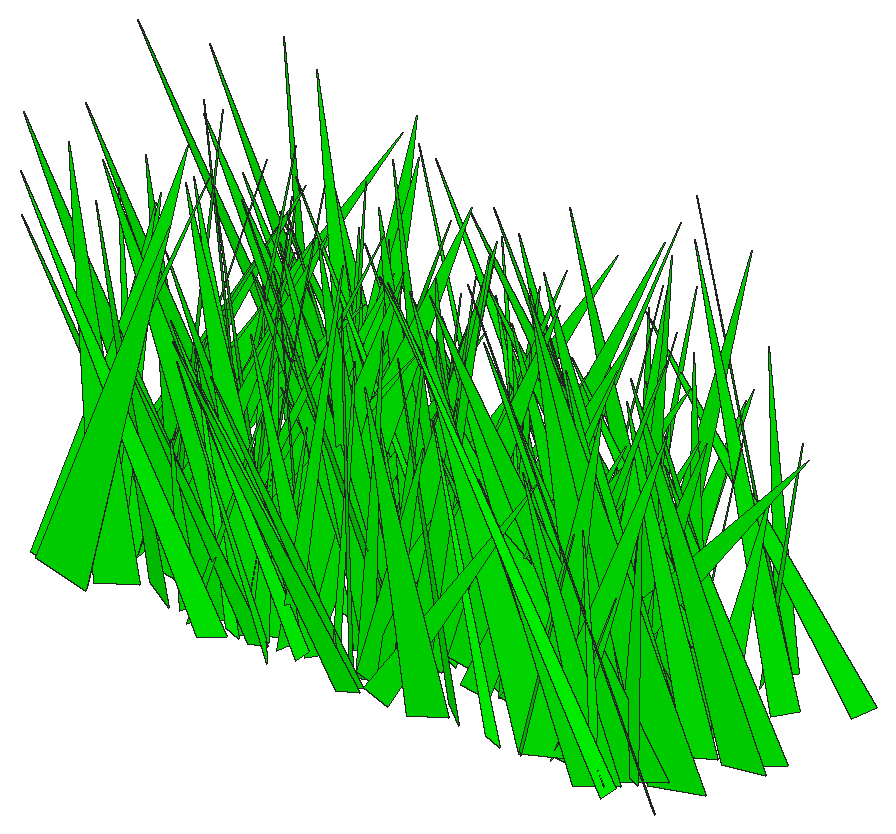
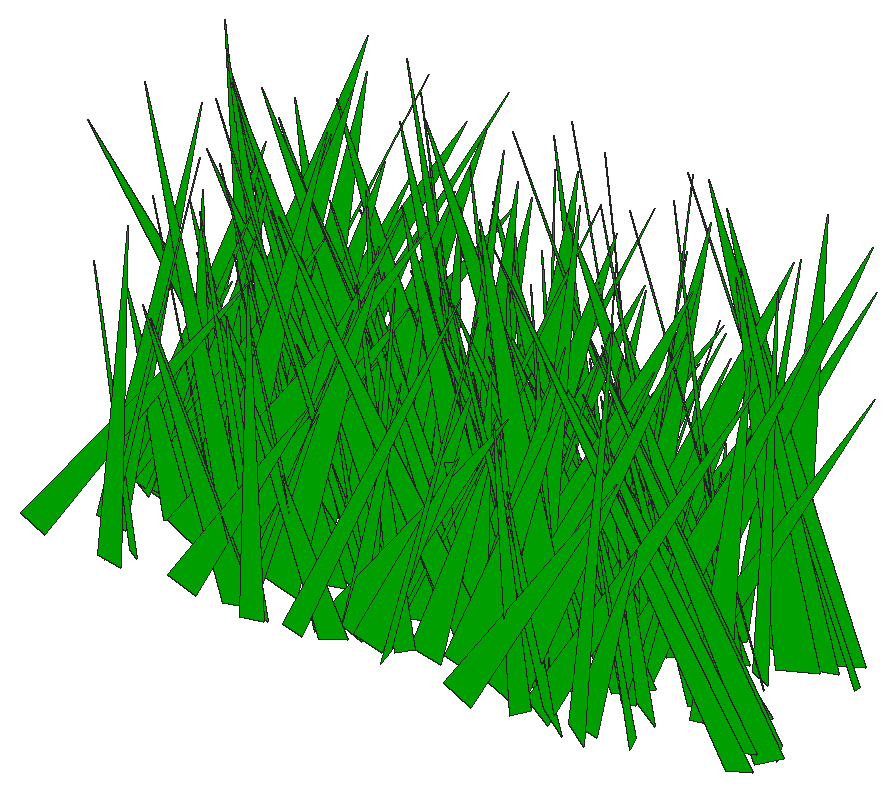
# SketchUp Ruby script. Lengths in inches.
U = 1.inch
M = Sketchup.active_model
def pt(a) = Geom::Point3d.new(a.map { |v| v * U })
def face(e, loops, mat)
  f = e.add_face(loops[0].map { |a| pt(a) })
  loops[1..].each { |l| e.add_face(l.map { |a| pt(a) }).erase! }
  f.material = f.back_material = mat if mat
  f
end
# faces: each face lists its corners as indices into pts; further lists are holes
def faces(e, pts, list, mat = nil) = list.each { |f| face(e, (f[0].is_a?(Array) ? f : [f]).map { |l| l.map { |i| pts[i] } }, mat) }
# xy, xz, yz: faces in a plane at the given z, y or x. An outline is a flat list of corners, or four numbers for a rectangle; further outlines are holes
def ring(l) = l.size == 4 ? [[l[0], l[1]], [l[2], l[1]], [l[2], l[3]], [l[0], l[3]]] : l.each_slice(2).to_a
def flat(e, list, mat, &to3) = list.each { |f| face(e, (f[0].is_a?(Array) ? f : [f]).map { |l| ring(l).map { |u, v| to3.(u, v) } }, mat) }
def xy(e, z, list, mat = nil) = flat(e, list, mat) { |x, y| [x, y, z] }
def xz(e, y, list, mat = nil) = flat(e, list, mat) { |x, z| [x, y, z] }
def yz(e, x, list, mat = nil) = flat(e, list, mat) { |y, z| [x, y, z] }
def lines(e, pts, list) = list.each { |a, b| e.add_line(pt(pts[a]), pt(pts[b])) }
# prism: a flat outline (further loops are holes) pulled along v
def prism(e, loops, v, mat = nil)
  f = face(e, loops, mat); d = Geom::Vector3d.new(v.map { |x| x * U })
  f.pushpull(f.normal.samedirection?(d) ? d.length : -d.length)
end
def box(e, o, s, mat = nil) = prism(e, [[o, [o[0] + s[0], o[1], o[2]], [o[0] + s[0], o[1] + s[1], o[2]], [o[0], o[1] + s[1], o[2]]]], [0, 0, s[2]], mat)
def at(x, y, z, deg = 0) = Geom::Transformation.translation(pt([x, y, z])) * Geom::Transformation.rotation(ORIGIN, Z_AXIS, deg.degrees)
def axes(o, x, y, z) = Geom::Transformation.new([*x, 0, *y, 0, *z, 0, *pt(o).to_a, 1])
def part(name) = M.definitions.add(name)
# library, detail: a bought-in or finely detailed component or shape, given as its bounding box
def library(name, o, s) = part(name).tap { |d| box(d.entities, o, s) }
def detail(e, o, s) = box(e.add_group.entities, o, s)
def put(e, d, t, mat = nil) = e.add_instance(d, t).tap { |i| i.material = mat if mat }
def group(e, t, mat = nil) = e.add_group.tap { |g| g.transformation = t; g.material = mat if mat }.entities
root = M.entities
M.materials.add("[0065_Lime]").color = [0, 255, 0]
c1 = part("fur_instance\#9")
p = [[0.8125,0,1.79],[0.67,-0.02,1.48],[0,-0.11,0],[0,0.11,0]]
faces(c1.entities,p,[[0,1,2,3]])
put(root,c1,axes([48.68,23.55,1.48],[-4.07372,-0.91201,0.20358],[6.33455,-0.56704,-1.2527],[1.43544,-0.08593,6.1059]),"[0065_Lime]")
put(root,c1,axes([51.56,20.1,1.48],[-5.89201,-0.44305,0.24837],[3.10748,-0.79083,1.50424],[-0.61473,0.24881,5.22342]),"[0065_Lime]")
put(root,c1,axes([46.21,23.61,1.48],[6.74369,-0.00029,0.17431],[0.06941,0.89987,-1.72693],[-0.20276,0.29849,5.20647]),"[0065_Lime]")
put(root,c1,axes([52.6875,25.88,1.48],[-7.7799,-0.6017,0.36466],[4.2396,-1.04797,1.90215],[-0.75013,0.31754,6.96855]),"[0065_Lime]")
put(root,c1,axes([51.88,23.01,1.48],[-4.98454,-0.94604,0.09844],[6.66124,-0.68968,1.06821],[-0.98445,0.12331,6.72962]),"[0065_Lime]")
put(root,c1,axes([49.63,19.33,1.48],[5.19849,-0.96659,1.66799],[6.54163,0.78443,1.74286],[-2.95466,0.03608,6.7934]),"[0065_Lime]")
put(root,c1,axes([49.17,20.73,1.48],[-6.82183,0.05565,2.74804],[-1.5285,-1.00055,-1.83157],[3.03877,-0.37835,5.24787]),"[0065_Lime]")
put(root,c1,axes([46.15,24.125,1.48],[6.47814,-0.51925,0.67202],[3.76421,0.85822,-1.78814],[0.41013,0.32493,5.79688]),"[0065_Lime]")
put(root,c1,axes([48.32,19.46,1.48],[-1.28615,1.01519,1.55532],[-7.2535,-0.23522,1.17596],[1.79941,-0.22254,5.85201]),"[0065_Lime]")
put(root,c1,axes([48.63,19.8,1.48],[-3.52804,0.92999,1.4678],[-6.38089,-0.54957,1.52025],[2.51841,-0.08963,5.90809]),"[0065_Lime]")
put(root,c1,axes([47.06,24.2,1.48],[3.35952,0.76991,0.39872],[-5.32449,0.43483,1.54786],[1.38223,-0.19626,4.99344]),"[0065_Lime]")
put(root,c1,axes([46.78,19.58,1.48],[8.93201,0.21826,0.83479],[-1.73967,1.2302,1.53789],[-0.66288,-0.28758,7.21231]),"[0065_Lime]")
put(root,c1,axes([47.96,18.92,1.48],[-2.61508,1.25456,1.37276],[-8.47503,-0.42576,2.3563],[3.27618,-0.09998,7.19117]),"[0065_Lime]")
put(root,c1,axes([53.14,19.56,1.48],[-4.27079,-1.12782,0.92461],[7.91508,-0.54119,2.06895],[-1.75029,0.30458,7.10002]),"[0065_Lime]")
put(root,c1,axes([49.6,25.65,1.48],[4.1549,0.03918,1.15757],[0.34748,0.56226,-1.46292],[-1.40791,0.25439,3.05505]),"[0065_Lime]")
put(root,c1,axes([50.97,24.03,1.48],[-4.48205,-0.3349,0.36033],[2.21663,-0.61916,-1.04063],[0.98144,-0.13104,3.99588]),"[0065_Lime]")
put(root,c1,axes([51.14,25.84,1.48],[0.00797,0.625,0.25599],[-4.29085,0.0131,-0.9836],[-1.21279,-0.04225,3.48166]),"[0065_Lime]")
put(root,c1,axes([53.42,18.66,1.48],[-7.20831,0.54493,0.08946],[-3.85095,-1.00106,-0.97205],[-0.47041,-0.15514,6.58667]),"[0065_Lime]")
put(root,c1,axes([50.88,19.57,1.48],[-6.81332,-0.57827,1.01934],[3.6731,-0.95369,-1.88538],[2.23932,-0.19513,6.19395]),"[0065_Lime]")
put(root,c1,axes([49.39,21.31,1.48],[4.09738,-0.2315,0.5266],[1.45263,0.57084,0.93058],[-1.01151,-0.11797,3.46956]),"[0065_Lime]")
put(root,c1,axes([48.13,18.79,1.48],[0.37992,-1.11269,1.4575],[7.83928,-0.01529,-1.74306],[2.11176,0.25693,6.2084]),"[0065_Lime]")
put(root,c1,axes([51.09,26.22,1.48],[-7.64642,-0.31284,2.79186],[3.21779,-1.09124,1.73359],[2.52646,0.44302,6.2417]),"[0065_Lime]")
put(root,c1,axes([46.45,25.04,1.48],[7.70161,0.7186,0.15562],[-4.98191,1.04168,1.94706],[1.17045,-0.29463,7.26346]),"[0065_Lime]")
put(root,c1,axes([50.32,24.19,1.48],[5.50694,0.53946,0.7244],[-3.39627,0.75869,-1.84981],[-1.99931,0.1971,5.13762]),"[0065_Lime]")
put(root,c1,axes([50.11,20.95,1.48],[8.62522,0.15611,2.42075],[-0.39976,1.25374,-1.76682],[-3.15138,0.26822,6.84963]),"[0065_Lime]")
put(root,c1,axes([53.9,25.77,1.48],[-6.69789,-0.79189,0.81059],[5.71052,-0.9106,1.41088],[-0.37651,0.27607,6.97887]),"[0065_Lime]")
put(root,c1,axes([49.07,20.81,1.48],[8.5082,0.29483,1.00981],[-1.81444,1.18877,-1.51533],[-1.62829,0.21588,6.96508]),"[0065_Lime]")
put(root,c1,axes([49.58,23.01,1.48],[5.62934,0.37435,1.24764],[-3.00109,0.76666,1.25101],[-0.66592,-0.29052,4.90896]),"[0065_Lime]")
put(root,c1,axes([54.51,19.54,1.48],[-2.83101,1.08435,1.40047],[-7.66821,-0.31393,-2.1111],[-1.92679,-0.34384,6.34401]),"[0065_Lime]")
put(root,c1,axes([47.75,22.59,1.48],[4.43363,0.75456,0.40978],[-4.86388,0.51978,2.74705],[2.33055,-0.35067,4.95359]),"[0065_Lime]")
put(root,c1,axes([51.97,19.51,1.48],[2.89859,-0.42098,0.0198],[2.6624,0.36412,1.53792],[-1.37392,-0.18255,3.02197]),"[0065_Lime]")
put(root,c1,axes([50.93,23.875,1.48],[-0.9214,-0.66428,0.38057],[4.40262,-0.14456,-1.40289],[1.78438,0.01367,3.65788]),"[0065_Lime]")
put(root,c1,axes([54.39,20.9,1.48],[-4.60535,-0.60324,0.97308],[4.44191,-0.60177,1.40869],[-0.36068,0.29139,4.92364]),"[0065_Lime]")
put(root,c1,axes([54.92,26.51,1.48],[-3.41391,-0.66832,0.40587],[4.55813,-0.42867,1.71429],[-1.44688,0.22646,4.44291]),"[0065_Lime]")
put(root,c1,axes([50.23,20.58,1.48],[3.70843,-0.68218,0.79021],[4.91564,0.48696,-1.17652],[0.59091,0.23032,4.82796]),"[0065_Lime]")
put(root,c1,axes([51.0625,21.53,1.48],[8.5129,0.07603,1.98454],[0.11365,1.20408,-1.86829],[-2.49646,0.31407,6.68221]),"[0065_Lime]")
put(root,c1,axes([53.85,20.47,1.48],[-6.25726,0.72762,0.42309],[-5.08217,-0.87895,0.92111],[1.12025,0.0767,6.54198]),"[0065_Lime]")
put(root,c1,axes([53.5625,21.07,1.48],[-7.52551,-0.2028,1.95223],[1.84318,-1.08667,0.91837],[2.10853,0.2261,6.16488]),"[0065_Lime]")
put(root,c1,axes([54.66,19.0625,1.48],[-3.79363,-0.52252,0.09486],[3.63146,-0.51499,1.03323],[-0.80852,0.13864,4.19565]),"[0065_Lime]")
put(root,c1,axes([53.5,20.51,1.48],[-8.88237,-0.10563,2.45717],[1.31519,-1.29059,1.28654],[2.82146,0.26906,7.13581]),"[0065_Lime]")
put(root,c1,axes([49.51,21.66,1.48],[4.14624,-1.01049,0.18664],[7.05449,0.56365,-1.43235],[1.41409,0.15094,6.59835]),"[0065_Lime]")
put(root,c1,axes([55.65,23.77,1.48],[1.72035,-1.18418,1.79479],[7.65245,0.35645,3.02737],[-4.16257,0.16588,6.30728]),"[0065_Lime]")
put(root,c1,axes([52.6,21.36,1.48],[-5.25279,0.17933,1.77712],[-0.64661,-0.77908,1.36978],[2.44618,0.17914,4.17818]),"[0065_Lime]")
put(root,c1,axes([55.3,24.21,1.48],[-5.86449,0.56431,0.65677],[-4.087,-0.79274,-1.32174],[-0.27545,-0.25201,5.62841]),"[0065_Lime]")
put(root,c1,axes([52.32,22.48,1.48],[5.06736,-0.33017,0.90518],[1.83122,0.69643,1.72939],[-1.84552,-0.21553,4.2014]),"[0065_Lime]")
put(root,c1,axes([53.72,19.14,1.48],[-4.9759,0.24562,0.70754],[-1.44297,-0.68805,1.28948],[1.31523,0.17437,4.09155]),"[0065_Lime]")
put(root,c1,axes([54.64,19.72,1.48],[-4.08934,0.93619,1.83139],[-7.03109,-0.55175,-0.93643],[0.1439,-0.35476,6.28938]),"[0065_Lime]")
put(root,c1,axes([52.75,25.39,1.48],[3.28564,0.43236,0.1437],[-2.92735,0.44916,-0.99859],[-0.96385,0.10969,3.52269]),"[0065_Lime]")
put(root,c1,axes([53.01,26.21,1.48],[-4.55212,0.46135,1.34669],[-2.83365,-0.67608,1.42368],[2.34329,0.07867,4.33771]),"[0065_Lime]")
put(root,c1,axes([51.19,23.29,1.48],[5.23543,-0.52675,1.25405],[4.0498,0.66505,-1.82574],[0.16874,0.3819,4.90915]),"[0065_Lime]")
put(root,c1,axes([54.26,24.32,1.48],[-7.64333,0.55072,2.8893],[-4.61776,-1.12251,-0.91296],[2.57949,-0.37765,6.92697]),"[0065_Lime]")
put(root,c1,axes([52.49,18.9,1.48],[4.931,0.28755,0.31731],[-1.83441,0.6661,-1.36568],[-0.98728,0.19854,4.12229]),"[0065_Lime]")
put(root,c1,axes([53.2,24.53,1.48],[7.03366,-0.09981,2.06156],[0.33102,1.04161,0.94262],[-2.61121,-0.13681,5.67259]),"[0065_Lime]")
put(root,c1,axes([54.08,23.84,1.48],[3.40113,0.86605,0.12271],[-5.88469,0.46326,-1.64257],[-1.83825,0.11935,5.48531]),"[0065_Lime]")
put(root,c1,axes([55.97,19.34,1.48],[-5.93388,0.1731,0.58285],[-1.38784,-0.79987,-1.38837],[0.32384,-0.25611,4.73006]),"[0065_Lime]")
put(root,c1,axes([55.375,24.26,1.48],[-7.51285,-0.23848,0.8594],[1.03209,-0.95713,-2.93037],[1.71214,-0.46949,5.53747]),"[0065_Lime]")
put(root,c1,axes([51.41,23.5625,1.48],[2.37957,-0.75187,0.75282],[5.1652,0.26959,-1.78006],[1.67556,0.23673,4.41823]),"[0065_Lime]")
put(root,c1,axes([55.04,18.95,1.48],[-6.26405,-0.20787,0.75441],[0.77039,-0.76463,-2.82752],[1.56687,-0.45508,4.40622]),"[0065_Lime]")
put(root,c1,axes([55.63,24.84,1.48],[-3.44068,0.83272,1.3114],[-6.13739,-0.45674,-0.93567],[-0.22393,-0.27651,5.49482]),"[0065_Lime]")
put(root,c1,axes([55.71,25.23,1.48],[-0.18513,-0.84445,1.39136],[5.99324,0.044,1.42243],[-1.76686,0.23773,4.67915]),"[0065_Lime]")
put(root,c1,axes([52.91,20.58,1.48],[8.57566,0.01759,2.28666],[-1.06979,1.19225,2.34711],[-2.6027,-0.43207,6.56961]),"[0065_Lime]")
put(root,c1,axes([55.45,21.82,1.48],[-5.96345,0.20557,0.72889],[-1.27422,-0.8357,1.00018],[1.14871,0.14019,4.89341]),"[0065_Lime]")
put(root,c1,axes([53.01,24.57,1.48],[-3.67742,1.08212,2.14408],[-7.58583,-0.60299,1.58919],[2.95091,-0.20155,6.75726]),"[0065_Lime]")
put(root,c1,axes([51.99,26.09,1.48],[8.60186,-0.31901,0.1036],[1.89633,1.0451,3.66035],[-1.2547,-0.60752,6.24245]),"[0065_Lime]")
put(root,c1,axes([53.45,23.76,1.48],[-2.351,1.20259,0.34889],[-8.26195,-0.3347,1.82297],[2.27354,0.02728,6.98538]),"[0065_Lime]")
put(root,c1,axes([54.59,19.24,1.48],[2.56597,0.4753,0.14337],[-3.17849,0.34864,-1.09065],[-1.17022,0.09525,3.27671]),"[0065_Lime]")
put(root,c1,axes([51.58,21.16,1.48],[4.61856,0.68681,0.07581],[-4.59644,0.60396,1.92972],[1.6646,-0.23788,5.1182]),"[0065_Lime]")
put(root,c1,axes([53.74,19.56,1.48],[8.65031,0.2378,1.91156],[-1.40778,1.25431,-1.01357],[-2.53076,0.11508,7.09766]),"[0065_Lime]")
put(root,c1,axes([51.87,20.18,1.48],[8.60319,0.32378,0.59859],[-2.38743,1.19803,0.9883],[-0.38879,-0.19198,7.17687]),"[0065_Lime]")
put(root,c1,axes([57.47,19.28,1.48],[-5.5116,0.08664,0.09538],[-0.61548,-0.71755,-1.69006],[-0.12301,-0.29191,4.18263]),"[0065_Lime]")
put(root,c1,axes([55.25,20.35,1.48],[-6.38234,-0.22789,1.89956],[0.52334,-0.88679,-2.40155],[2.79463,-0.35439,4.78793]),"[0065_Lime]")
put(root,c1,axes([58.14,18.59,1.48],[-4.46139,-0.61599,0.07032],[4.19664,-0.59489,1.54199],[-1.27,0.19814,4.84835]),"[0065_Lime]")
put(root,c1,axes([54.5,20.0625,1.48],[4.39427,-0.2447,0.54564],[1.44022,0.59803,1.3129],[-1.18675,-0.18032,3.6137]),"[0065_Lime]")
put(root,c1,axes([56.29,19.61,1.48],[4.01222,-0.58925,1.74626],[3.71943,0.6394,1.57555],[-2.89128,0.00485,4.45011]),"[0065_Lime]")
put(root,c1,axes([54.96,24.15,1.48],[5.44446,-0.70671,0.71722],[4.68225,0.76325,1.68406],[-2.03665,-0.13448,5.78895]),"[0065_Lime]")
put(root,c1,axes([56.39,22.37,1.48],[-5.33871,-0.21661,0.6979],[1.16277,-0.721,-1.61358],[1.32683,-0.23974,4.22216]),"[0065_Lime]")
put(root,c1,axes([52.625,22.68,1.48],[3.73456,-0.72986,0.04607],[4.97073,0.4993,-1.54212],[1.50776,0.1617,4.96988]),"[0065_Lime]")
put(root,c1,axes([57.28,21.96,1.48],[-2.74332,-0.5244,1.46229],[4.07936,-0.28938,1.58614],[-0.71954,0.3587,3.41735]),"[0065_Lime]")
put(root,c1,axes([58.14,18.88,1.48],[-4.59668,-0.41679,0.18808],[2.89229,-0.61203,1.32268],[-0.69693,0.20899,4.2487]),"[0065_Lime]")
put(root,c1,axes([58.01,21.79,1.48],[-1.89388,-0.60808,0.13044],[4,-0.23623,1.52448],[-1.65893,0.1246,3.52693]),"[0065_Lime]")
put(root,c1,axes([57.45,22.69,1.48],[0.95097,0.82668,0.96773],[-5.55583,0.18529,-1.69157],[-2.27137,-0.10711,4.54279]),"[0065_Lime]")
put(root,c1,axes([56.94,25.34,1.48],[0.29135,-0.66137,0.80496],[4.62326,0.07691,1.01039],[-1.32577,0.12287,3.70035]),"[0065_Lime]")
put(root,c1,axes([57.7,26.09,1.48],[-7.68937,0.13821,1.08137],[-0.6827,-1.07452,1.39008],[1.50624,0.21855,6.15047]),"[0065_Lime]")
put(root,c1,axes([58.48,20.36,1.48],[-2.70343,-0.85811,1.74048],[6.26499,-0.26557,2.05102],[-1.61908,0.40519,5.03026]),"[0065_Lime]")
put(root,c1,axes([55.18,23.13,1.48],[5.05954,0.14031,0.9721],[-0.63844,0.70755,-1.22342],[-1.42042,0.18174,4.0125]),"[0065_Lime]")
put(root,c1,axes([53.97,21.32,1.48],[3.79076,-0.90093,1.32915],[6.59534,0.49341,-1.23862],[0.52788,0.30496,5.93056]),"[0065_Lime]")
put(root,c1,axes([56.05,24.56,1.48],[3.74877,-0.6663,0.11044],[4.41637,0.4991,1.71313],[-1.73149,-0.16956,4.60866]),"[0065_Lime]")
put(root,c1,axes([58.73,24.23,1.48],[-6.64891,0.12481,0.04581],[-0.84838,-0.90682,1.32009],[0.26907,0.22503,5.29426]),"[0065_Lime]")
put(root,c1,axes([58.38,20,1.48],[1.90382,0.98367,2.08815],[-6.78027,0.38329,-1.96017],[-3.10209,-0.23406,5.56592]),"[0065_Lime]")
put(root,c1,axes([59.69,19.52,1.48],[-8.71029,-0.2024,0.74735],[1.66915,-1.15126,2.42354],[0.36455,0.43512,6.75999]),"[0065_Lime]")
put(root,c1,axes([55.32,19.51,1.48],[7.82658,-0.38735,1.34895],[2.3529,1.10727,1.62181],[-2.19383,-0.19434,6.55183]),"[0065_Lime]")
put(root,c1,axes([55.94,22.37,1.48],[4.078,0.20173,0.54797],[-1.10512,0.54883,-1.32872],[-1.13731,0.19002,3.25596]),"[0065_Lime]")
put(root,c1,axes([53.71,22.63,1.48],[6.10895,-0.41429,0.2331],[2.92042,0.82689,-1.39384],[0.49575,0.23398,5.33859]),"[0065_Lime]")
put(root,c1,axes([59.67,25.45,1.48],[-1.34794,0.88752,0.30044],[-5.6979,-0.14722,-2.34099],[-2.75018,-0.12998,4.70286]),"[0065_Lime]")
put(root,c1,axes([59.56,22.3,1.48],[-9.16661,-0.12978,0.67653],[0.58146,-1.21657,-2.60761],[1.0985,-0.43904,7.02569]),"[0065_Lime]")
put(root,c1,axes([57.6,20.7,1.48],[1.78212,-1.1956,0.20242],[8.36483,0.2526,1.26816],[-1.57676,-0.01126,6.95646]),"[0065_Lime]")
put(root,c1,axes([54.23,21.47,1.48],[2.98922,1.21225,1.38029],[-8.62039,0.35452,1.91863],[1.73021,-0.32803,7.17452]),"[0065_Lime]")
put(root,c1,axes([58.5625,25.78,1.48],[-1.20662,0.58689,1.12083],[-4.23051,-0.09999,-1.25896],[-1.20246,-0.23715,3.30458]),"[0065_Lime]")
put(root,c1,axes([55.42,23.3,1.48],[6.21657,0.14176,1.00032],[-1.2912,0.85686,1.24017],[-0.92895,-0.24233,4.97041]),"[0065_Lime]")
put(root,c1,axes([55.91,22.69,1.48],[5.24544,0.31507,1.55132],[-2.866,0.67158,1.84125],[-0.67156,-0.40508,4.25924]),"[0065_Lime]")
put(root,c1,axes([58.1875,22.27,1.48],[3.19103,-1.07245,1.47914],[7.51375,0.49713,1.35299],[-2.25838,0.13862,6.59145]),"[0065_Lime]")
put(root,c1,axes([57.47,18.84,1.48],[-5.77678,0.17725,1.99881],[-0.344,-0.84039,1.83942],[2.74065,0.26813,4.44399]),"[0065_Lime]")
put(root,c1,axes([55.65,23.74,1.48],[1.38855,-1.11739,0.47627],[7.81643,0.17426,-1.37789],[1.57462,0.1203,6.41987]),"[0065_Lime]")
put(root,c1,axes([60.6,26.49,1.48],[-7.76787,0.27864,0.82332],[-2.18155,-1.05565,-1.64659],[0.44428,-0.31184,6.3098]),"[0065_Lime]")
put(root,c1,axes([59.01,21.84,1.48],[-7.29422,-0.57402,2.89469],[5.01932,-1.03167,1.51315],[2.03919,0.48609,6.62982]),"[0065_Lime]")
put(root,c1,axes([57.82,19.12,1.48],[6.88096,-0.08889,2.42439],[-0.24163,1.01523,1.70101],[-3.03731,-0.28214,5.35709]),"[0065_Lime]")
put(root,c1,axes([58.67,21.08,1.48],[-4.58879,-0.0268,1.10248],[-0.1409,-0.65353,-0.92035],[1.36145,-0.15796,3.62067]),"[0065_Lime]")
put(root,c1,axes([59.43,23.37,1.48],[-1.88293,0.6266,0.90988],[-4.55097,-0.22996,-0.92452],[-0.65171,-0.20452,3.82723]),"[0065_Lime]")
put(root,c1,axes([58.06,19.39,1.48],[5.36594,0.52664,1.50452],[-3.49094,0.79733,-1.11449],[-2.29807,0.01849,5.20602]),"[0065_Lime]")
put(root,c1,axes([57.83,21.9,1.48],[-6.28395,0.12673,2.66634],[0.34139,-0.93957,2.02882],[3.38259,0.33027,4.74858]),"[0065_Lime]")
put(root,c1,axes([59.5,25.36,1.48],[-5.28024,0.39538,0.28902],[-2.60097,-0.71716,1.43483],[1.13065,0.1967,4.65046]),"[0065_Lime]")
put(root,c1,axes([55.05,24.99,1.48],[4.46324,0.97602,0.25574],[-6.71083,0.59097,1.91495],[1.8191,-0.21458,6.43695]),"[0065_Lime]")
put(root,c1,axes([57.52,25.5,1.48],[-4.75241,-0.62531,1.83856],[3.68448,-0.73537,-2.07931],[3.36693,-0.07789,4.87054]),"[0065_Lime]")
put(root,c1,axes([59.47,24.65,1.48],[-6.83993,0.29806,1.37285],[-1.49029,-0.95119,2.00729],[2.26425,0.27433,5.4683]),"[0065_Lime]")
put(root,c1,axes([58.83,22.5,1.48],[-3.92,-0.94741,0.50546],[6.55628,-0.55632,-1.2993],[1.691,-0.03929,6.20933]),"[0065_Lime]")
put(root,c1,axes([56.84,21.09,1.48],[2.63384,0.60764,0.72768],[-4.29637,0.3188,1.36859],[1.0203,-0.22615,3.88448]),"[0065_Lime]")
put(root,c1,axes([57.11,21.81,1.48],[4.11576,0.95837,2.65949],[-7.56093,0.5078,1.61009],[0.19564,-0.53636,6.27633]),"[0065_Lime]")
put(root,c1,axes([56.85,23.59,1.48],[7.51656,-0.21369,0.99577],[1.74935,1.04101,-1.25108],[-0.86664,0.24793,6.1112]),"[0065_Lime]")
put(root,c1,axes([58.37,19.34,1.48],[-1.52676,-0.77497,0.45076],[5.19475,-0.22823,-1.50665],[1.93335,0.00124,4.40419]),"[0065_Lime]")
put(root,c1,axes([58.97,19.02,1.48],[6.32929,0.45924,1.47279],[-2.99171,0.92275,-1.13491],[-2.23815,0.06527,5.68194]),"[0065_Lime]")
put(root,c1,axes([60.22,22.15,1.48],[-5.73575,-0.5586,0.54921],[3.53778,-0.77631,-2.01237],[1.93476,-0.23652,5.30788]),"[0065_Lime]")
put(root,c1,axes([58.66,21.81,1.48],[-4.13862,0.79566,0.19526],[-4.8001,-0.51431,2.91141],[3.01319,0.27354,4.90615]),"[0065_Lime]")
put(root,c1,axes([60.67,18.84,1.48],[2.7235,-0.91953,0.18068],[6.22014,0.37391,1.72914],[-2.04498,-0.08734,5.50009]),"[0065_Lime]")
put(root,c1,axes([59.26,20.15,1.48],[7.78698,0.25588,2.18233],[-2.27198,1.13029,0.92289],[-2.31352,-0.24872,6.43913]),"[0065_Lime]")
put(root,c1,axes([59.55,24.47,1.48],[3.77321,-0.24159,0.0667],[1.54213,0.48682,1.36579],[-0.76458,-0.21038,3.08388]),"[0065_Lime]")
put(root,c1,axes([60.91,22.2,1.48],[-5.11621,-0.64968,0.27547],[4.28012,-0.6892,-1.87097],[1.78093,-0.21001,5.28789]),"[0065_Lime]")
put(root,c1,axes([61.11,19.4,1.48],[-6.53289,-0.39913,1.19029],[2.2973,-0.91201,-1.90514],[2.22076,-0.23069,5.47234]),"[0065_Lime]")
put(root,c1,axes([59.18,20.04,1.48],[7.26992,0.62552,2.32608],[-4.98728,1.03817,0.95807],[-1.76662,-0.3567,6.86747]),"[0065_Lime]")
put(root,c1,axes([62.61,24.78,1.48],[-0.24328,1.06256,0.81538],[-7.31562,0.00741,-1.76776],[-2.16025,-0.14476,5.89465]),"[0065_Lime]")
put(root,c1,axes([57.66,21.76,1.48],[6.15095,0.51559,0.04633],[-3.61981,0.8499,1.03368],[0.60292,-0.1574,5.73342]),"[0065_Lime]")
put(root,c1,axes([60.9,23.58,1.48],[4.0925,-0.75162,0.18891],[4.94206,0.54612,1.97324],[-2.05944,-0.18308,5.11061]),"[0065_Lime]")
put(root,c1,axes([58.44,21.16,1.48],[3.84947,-1.04216,1.15776],[7.46668,0.4916,-1.59785],[1.1313,0.30153,6.60644]),"[0065_Lime]")
put(root,c1,axes([59.44,26.18,1.48],[1.12985,-0.63637,0.90802],[4.46052,0.10023,-1.31846],[1.36364,0.19941,3.56038]),"[0065_Lime]")
put(root,c1,axes([62.63,25.57,1.48],[-6.07982,-0.36186,0.32027],[2.30276,-0.81218,-1.82629],[1.21819,-0.27073,5.05069]),"[0065_Lime]")
put(root,c1,axes([64.76,24.59,1.48],[-4.7124,0.72277,0.78458],[-4.99735,-0.56734,-2.34608],[-1.55362,-0.36738,5.1666]),"[0065_Lime]")
put(root,c1,axes([60.26,25.9,1.48],[6.75589,0.10178,1.27084],[-0.38771,0.95588,-1.20167],[-1.67789,0.18895,5.3946]),"[0065_Lime]")
put(root,c1,axes([65.54,20.625,1.48],[-6.51871,0.72778,0.10628],[-4.95856,-0.86785,-2.0904],[-1.50158,-0.29364,6.4416]),"[0065_Lime]")
put(root,c1,axes([58.17,23.84,1.48],[7.74321,-0.75815,0.49336],[5.42162,1.07174,-1.1121],[0.29084,0.20616,7.59567]),"[0065_Lime]")
put(root,c1,axes([64.58,24.29,1.48],[-7.07232,-0.62189,0.78877],[4.52852,-0.96244,1.43801],[-0.14077,0.28264,6.63215]),"[0065_Lime]")
put(root,c1,axes([58.9,18.8125,1.48],[4.91546,-0.45524,0.53089],[3.21512,0.62068,-1.86132],[0.7649,0.31662,4.41209]),"[0065_Lime]")
put(root,c1,axes([62.87,18.88,1.48],[-5.61123,0.25907,0.57022],[-1.603,-0.77203,1.31681],[1.14937,0.18806,4.62033]),"[0065_Lime]")
put(root,c1,axes([58.84,25,1.48],[9.01433,0.2983,1.1324],[-2.40059,1.23636,1.73031],[-0.82575,-0.33786,7.33154]),"[0065_Lime]")
put(root,c1,axes([65.88,24.36,1.48],[-4.86516,-0.99642,0.72788],[6.77625,-0.59468,2.68861],[-2.27287,0.3599,6.45766]),"[0065_Lime]")
put(root,c1,axes([64.0625,20.72,1.48],[2.11869,-0.86064,2.81147],[6.16644,0.47123,1.75912],[-3.38148,0.3201,4.96946]),"[0065_Lime]")
put(root,c1,axes([61.83,20.92,1.48],[4.98115,0.63273,1.35023],[-4.32361,0.73757,-1.02825],[-2.08261,-0.01788,5.36416]),"[0065_Lime]")
put(root,c1,axes([64.41,19.1,1.48],[-3.8923,0.98121,1.50469],[-7.17161,-0.48951,-1.5781],[-0.86565,-0.3565,6.3083]),"[0065_Lime]")
put(root,c1,axes([61.81,26.7,1.48],[-4.17099,-0.63594,1.40073],[4.33184,-0.63276,-1.09189],[2.16393,0.04091,4.88572]),"[0065_Lime]")
put(root,c1,axes([64.44,26.41,1.48],[-2.2496,0.59803,0.82373],[-4.13612,-0.23862,-1.66856],[-1.42511,-0.25146,3.54239]),"[0065_Lime]")
put(root,c1,axes([61.26,23.95,1.48],[0.49299,-0.64179,0.38084],[4.45949,0.0512,-0.92844],[1.09204,0.08066,3.61951]),"[0065_Lime]")
put(root,c1,axes([61.4375,21.89,1.48],[4.26948,0.06121,0.43324],[-0.14504,0.53989,-1.61021],[-0.6726,0.27211,3.09733]),"[0065_Lime]")
put(root,c1,axes([59.3,21.71,1.48],[4.7068,-1.02079,0.31618],[7.11678,0.6326,-1.65958],[1.5086,0.2006,6.84257]),"[0065_Lime]")
put(root,c1,axes([65.68,23.34,1.48],[-5.54683,-0.29595,0.0377],[1.88893,-0.69057,2.22543],[-0.93277,0.36147,4.28245]),"[0065_Lime]")
put(root,c1,axes([65.07,19.74,1.48],[-1.74449,-0.70832,0.80679],[4.80809,-0.17325,1.78186],[-1.80986,0.22249,3.95607]),"[0065_Lime]")
put(root,c1,axes([64.2,20.86,1.48],[2.13514,0.85992,0.5937],[-5.65212,0.31649,-1.91152],[-2.45693,0.01922,4.91335]),"[0065_Lime]")
put(root,c1,axes([61.66,26.44,1.48],[7.1241,-0.20094,1.26803],[1.07848,1.00701,1.33835],[-1.81989,-0.18985,5.75691]),"[0065_Lime]")
put(root,c1,axes([60.77,21.32,1.48],[3.8804,0.63476,0.8645],[-4.55965,0.48529,1.60137],[0.86338,-0.29002,4.57165]),"[0065_Lime]")
put(root,c1,axes([60.8,20.69,1.48],[6.68567,-0.47348,1.02929],[3.58155,0.91238,-1.32825],[-0.35743,0.28591,5.94324]),"[0065_Lime]")
put(root,c1,axes([67.04,18.59,1.48],[-9.01603,0.18376,0.18695],[-1.32779,-1.2468,-1.30159],[-0.00585,-0.22716,7.2953]),"[0065_Lime]")
put(root,c1,axes([65.4,23.57,1.48],[-5.76064,-0.84105,2.52081],[6.72362,-0.75709,1.70186],[0.47081,0.52124,6.53936]),"[0065_Lime]")
put(root,c1,axes([60.1,22.45,1.48],[2.09079,-0.9909,1.46457],[6.69644,0.1588,-2.72482],[2.85084,0.35371,5.32631]),"[0065_Lime]")
put(root,c1,axes([65.53,20.93,1.48],[-1.68207,0.95417,2.09547],[-7.14365,-0.15039,-1.49937],[-1.30915,-0.40533,5.48923]),"[0065_Lime]")
put(root,c1,axes([61.8,20.85,1.48],[3.62019,-0.28819,0.00056],[1.97576,0.49,-0.90889],[0.55021,0.13666,3.26011]),"[0065_Lime]")
put(root,c1,axes([62.22,23.23,1.48],[7.22034,0.11811,1.1316],[-0.6082,1.02178,-1.00606],[-1.50731,0.15349,5.82657]),"[0065_Lime]")
put(root,c1,axes([67.39,19.69,1.48],[-2.17101,-1.16554,1.37289],[7.92821,-0.19422,2.76984],[-2.96525,0.33405,6.4006]),"[0065_Lime]")
put(root,c1,axes([66.37,20.78,1.48],[-5.94084,0.58027,1.74333],[-4.65153,-0.73055,-2.33963],[-0.09741,-0.50385,5.40005]),"[0065_Lime]")
put(root,c1,axes([61.88,23.4,1.48],[3.96856,0.56892,0.33376],[-4.02202,0.53607,1.02239],[0.61989,-0.16411,4.49679]),"[0065_Lime]")
put(root,c1,axes([62.54,26.32,1.48],[1.09917,0.75904,0.68039],[-5.33613,0.12301,1.10518],[1.18501,-0.15013,4.34556]),"[0065_Lime]")
put(root,c1,axes([63.95,24.21,1.48],[-2.34746,0.66771,0.17833],[-4.60966,-0.32779,0.97868],[1.17421,0.04805,4.19855]),"[0065_Lime]")
put(root,c1,axes([62.78,26.03,1.48],[0.2594,0.7763,0.14605],[-5.36721,0.02934,1.08226],[1.32159,-0.03324,4.36662]),"[0065_Lime]")
put(root,c1,axes([65.36,20.76,1.48],[1.70892,-1.18411,1.42828],[8.36817,0.28748,1.36161],[-2.01672,0.18947,6.86014]),"[0065_Lime]")
put(root,c1,axes([66.375,18.57,1.48],[-0.16337,0.71651,1.43758],[-4.97814,0.07592,-1.64236],[-2.08375,-0.23756,3.81093]),"[0065_Lime]")
put(root,c1,axes([63.81,18.86,1.48],[4.54167,0.09194,0.86915],[-0.30152,0.62819,-1.18426],[-1.21611,0.18761,3.53953]),"[0065_Lime]")
put(root,c1,axes([62.15,21.84,1.48],[7.84188,-0.37466,0.26559],[2.54545,1.08168,1.40301],[-0.85802,-0.2152,6.58959]),"[0065_Lime]")
put(root,c1,axes([66.97,21.06,1.48],[-3.0764,1.06385,2.32044],[-8.04006,-0.35416,-1.61174],[-0.90245,-0.47131,6.44894]),"[0065_Lime]")
put(root,c1,axes([63.22,25.21,1.48],[7.02118,0.66494,2.39995],[-5.46622,0.95256,1.73712],[-1.10362,-0.48774,6.66445]),"[0065_Lime]")
put(root,c1,axes([63.87,19.72,1.48],[-1.4639,-0.98517,1.23132],[6.87452,-0.25465,-1.41963],[2.04624,0.15071,5.65024]),"[0065_Lime]")
put(root,c1,axes([68.53,18.65,1.48],[-9.33153,-0.04843,0.4451],[0.47906,-1.26478,2.03367],[0.43443,0.35441,7.31825]),"[0065_Lime]")
put(root,c1,axes([64.15,21.84,1.48],[7.79963,-0.39671,2.61161],[3.56314,1.12188,-1.33023],[-2.36288,0.38224,6.61473]),"[0065_Lime]")
put(root,c1,axes([68.36,22.92,1.48],[-5.60688,0.55266,0.35217],[-3.87389,-0.74524,-1.61846],[-0.80575,-0.26278,5.33061]),"[0065_Lime]")
put(root,c1,axes([66.68,18.86,1.48],[1.55881,-0.7213,1.63146],[5.07502,0.30206,1.26669],[-2.14851,0.19018,4.17575]),"[0065_Lime]")
put(root,c1,axes([67.25,26.24,1.48],[-8.5569,-0.11092,1.70478],[1.27466,-1.19757,1.62223],[1.84142,0.31355,6.79899]),"[0065_Lime]")
put(root,c1,axes([63.63,23.43,1.48],[-2.29516,-0.89648,0.38462],[5.61324,-0.31607,-2.52364],[3.06878,-0.09235,4.90376]),"[0065_Lime]")
put(root,c1,axes([64.86,22.35,1.48],[-6.77292,-0.70082,3.22903],[5.00344,-1.08877,-0.97457],[3.94955,0.17748,6.77195]),"[0065_Lime]")
put(root,c1,axes([67.12,20.59,1.48],[-0.13581,-0.97625,1.6684],[7.07453,0.04411,1.24593],[-1.55766,0.28546,5.51327]),"[0065_Lime]")
put(root,c1,axes([64.7,19.25,1.48],[4.08507,-0.13368,0.16844],[0.83826,0.54675,1.08927],[-0.49522,-0.17724,3.23321]),"[0065_Lime]")
put(root,c1,axes([69.66,26.28,1.48],[-6.48893,0.46195,0.14723],[-3.09763,-0.8375,-2.27584],[-1.11583,-0.36143,5.46173]),"[0065_Lime]")
put(root,c1,axes([68.38,19.86,1.48],[-1.04396,-1.28864,0.99078],[9.02186,-0.1037,1.77021],[-2.04717,0.20015,7.29605]),"[0065_Lime]")
put(root,c1,axes([67.65,22.91,1.48],[-3.51473,0.64251,1.1681],[-4.79169,-0.466,-0.95033],[-0.09755,-0.25977,4.59387]),"[0065_Lime]")
put(root,c1,axes([67,22.46,1.48],[6.25662,0.85331,0.22888],[-4.89949,0.74139,-4.00633],[-3.59878,0.47417,5.85224]),"[0065_Lime]")
put(root,c1,axes([66.42,18.86,1.48],[-4.48271,0.09085,1.81153],[-1.28964,-0.66371,-0.99612],[1.92735,-0.2328,3.5468]),"[0065_Lime]")
put(root,c1,axes([64.52,19.27,1.48],[4.79654,-0.74615,1.23746],[5.52301,0.64369,-1.15875],[0.0814,0.29264,5.70395]),"[0065_Lime]")
put(root,c1,axes([67.77,21.65,1.48],[3.36418,-0.64982,2.48304],[4.72582,0.59849,1.01199],[-2.89322,0.22198,4.54023]),"[0065_Lime]")
put(root,c1,axes([68.03,24.94,1.48],[-7.79453,0.40604,2.3394],[-3.57244,-1.10037,-1.4757],[1.96439,-0.39002,6.59883]),"[0065_Lime]")
put(root,c1,axes([66.77,26.6,1.48],[-5.39657,0.28238,2.59602],[-2.99746,-0.79627,-1.22044],[2.28896,-0.37699,4.52233]),"[0065_Lime]")
put(root,c1,axes([68.66,22.9,1.48],[-5.67562,-0.40587,1.08521],[3.16019,-0.76357,1.36608],[0.36868,0.29691,4.9967]),"[0065_Lime]")
put(root,c1,axes([62.76,22.29,1.48],[4.54498,-0.85618,0.20104],[5.52694,0.56006,-2.74761],[2.57663,0.30889,5.53908]),"[0065_Lime]")
put(root,c1,axes([66.17,22.8,1.48],[5.74123,0.17202,1.11451],[-0.95778,0.81924,-0.97263],[-1.56801,0.12944,4.67486]),"[0065_Lime]")
put(root,c1,axes([66.85,19.7,1.48],[-4.09685,-0.54206,1.37729],[3.51055,-0.62273,-1.30361],[2.329,-0.01486,4.38768]),"[0065_Lime]")
put(root,c1,axes([69.0625,21.87,1.48],[-2.07115,-0.97895,0.7107],[6.94927,-0.26752,1.05175],[-1.00331,0.16795,5.81766]),"[0065_Lime]")
put(root,c1,axes([66.68,23.74,1.48],[-1.05444,0.66318,0.30368],[-4.56582,-0.15666,0.97464],[1.25172,-0.01278,3.81093]),"[0065_Lime]")
put(root,c1,axes([66.51,25.89,1.48],[5.25945,-0.12182,0.98153],[0.46969,0.72803,1.36246],[-1.40961,-0.21193,4.11621]),"[0065_Lime]")
put(root,c1,axes([69.51,22.51,1.48],[0.05986,0.77979,0.2265],[-5.04335,0.02405,-1.89242],[-2.33203,-0.03199,4.09844]),"[0065_Lime]")
